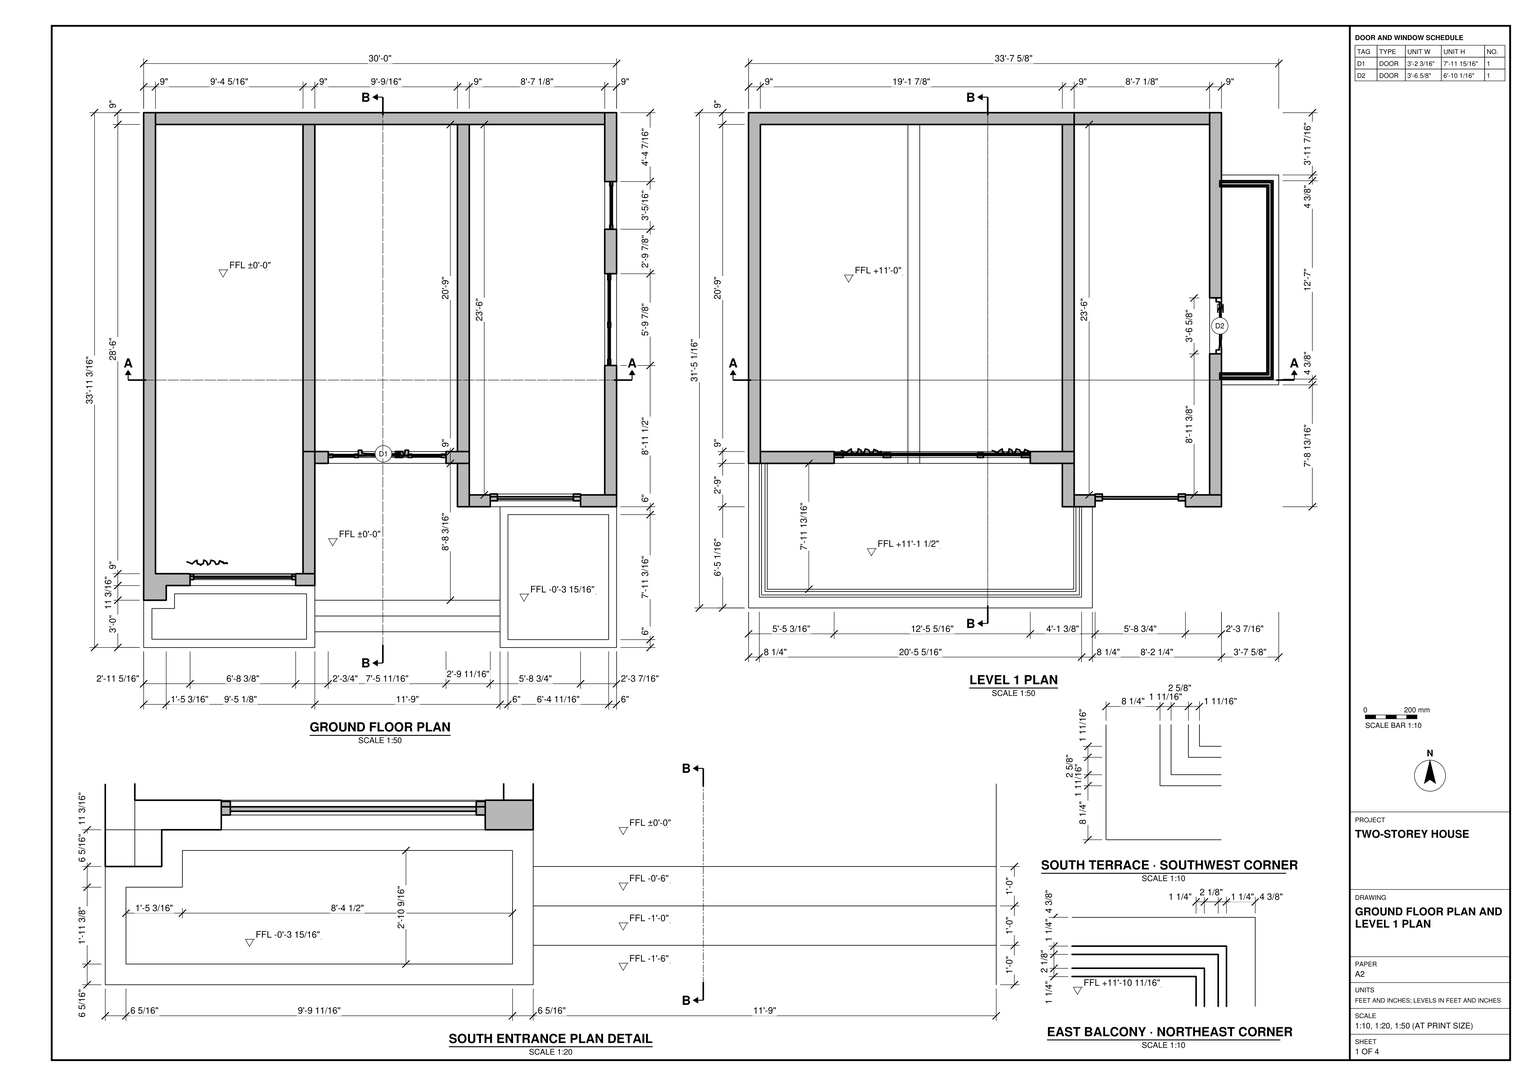
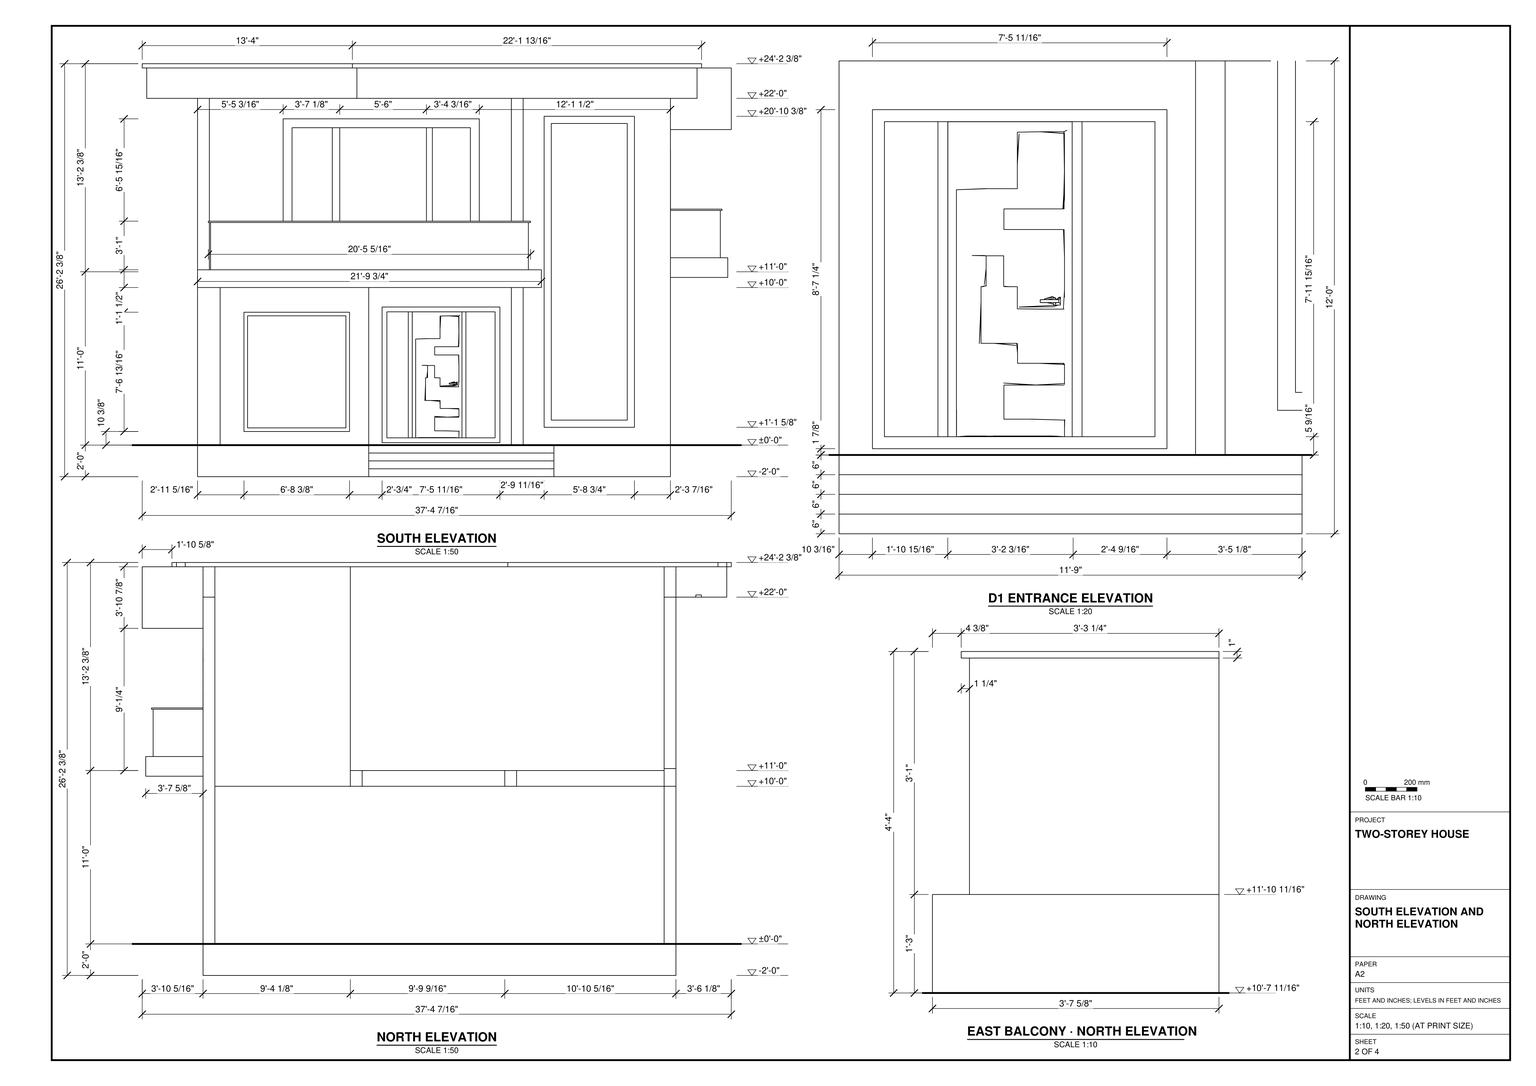
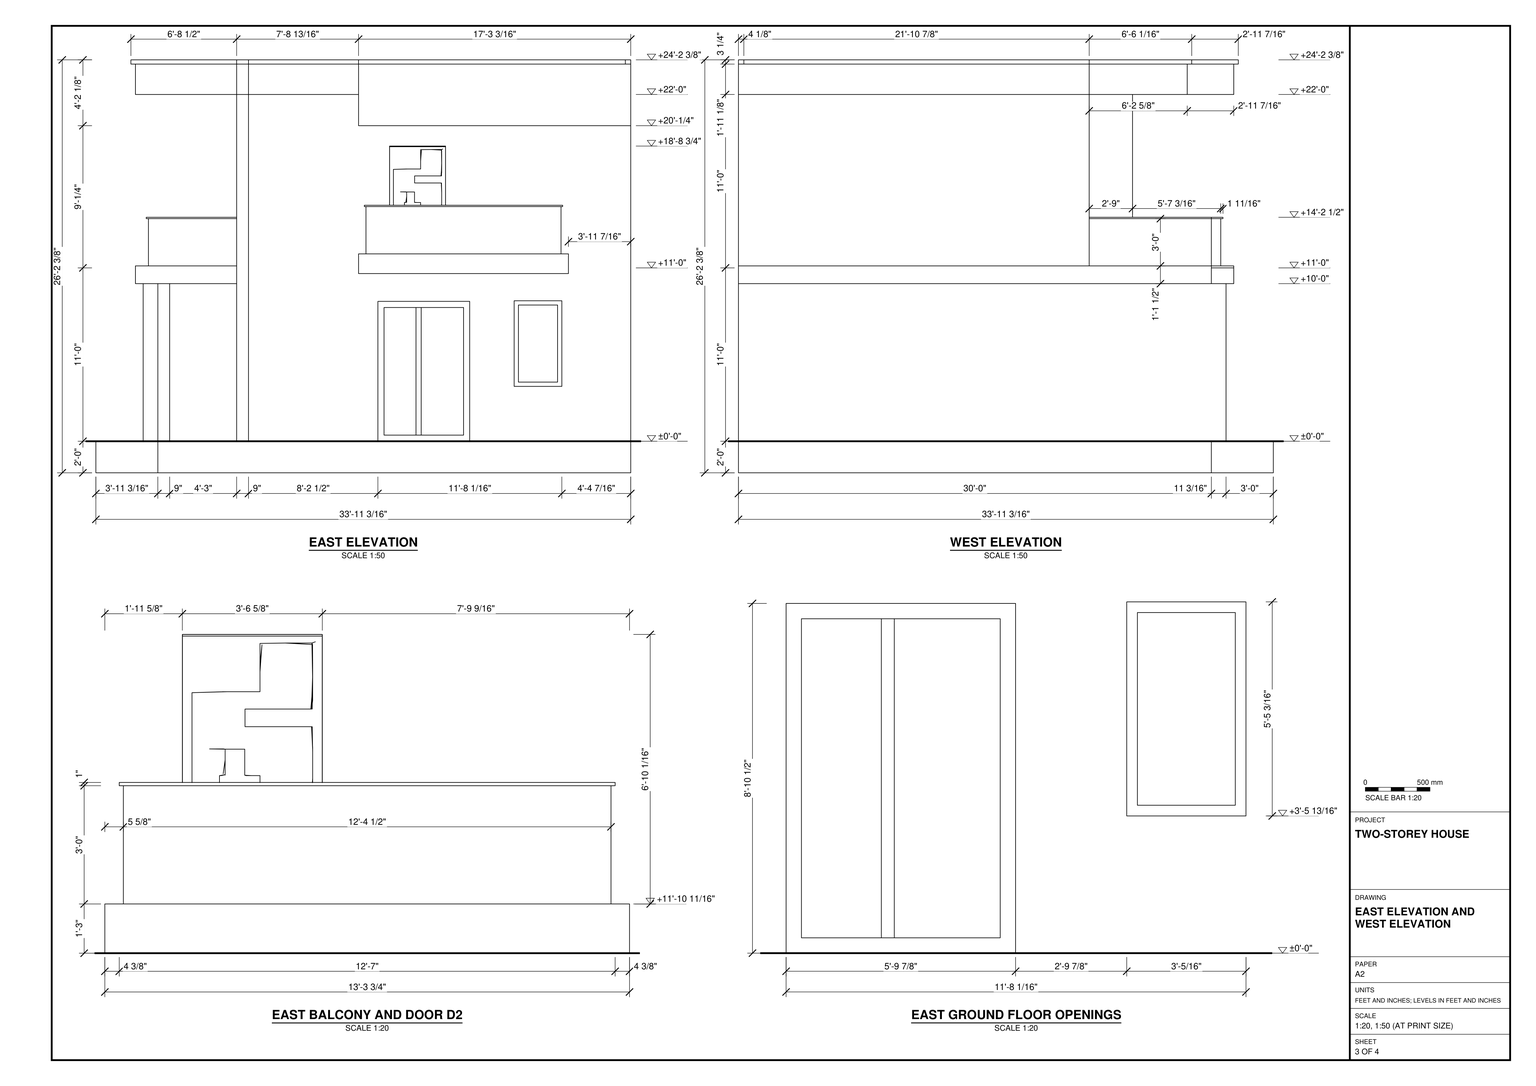
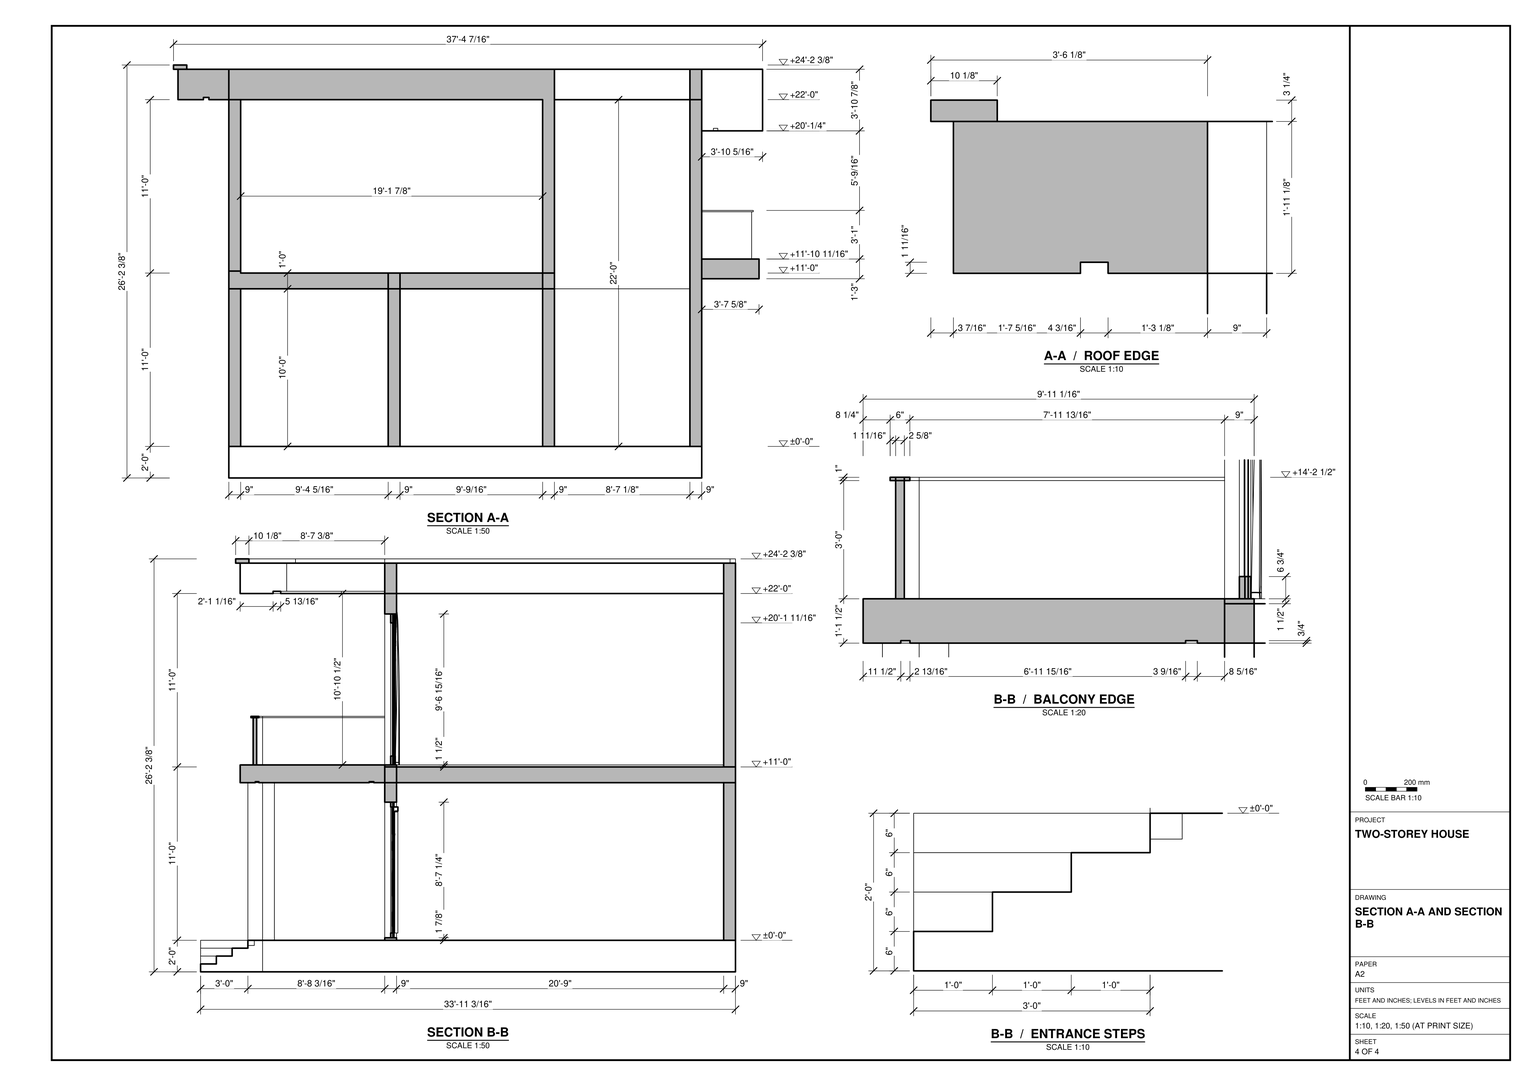
Build the house in SketchUp from task_files/diagram_01.pdf. Work in feet and inches. The overall model extents are 37'-4 7/16" east to west, 33'-11 3/16" north to south and 26'-2 3/8" from the bottom of the base to the top of the roof. Set the ground floor at ±0'-0" and the upper floor at +11'-0".

Use the plans to lay out the base, floor slabs and walls. Follow the 9" wall thicknesses where indicated. On the ground floor, run the partitions north to south and set the central entrance back between the flanking bays. Model the broad approach steps, entrance door and side panels. On the upper floor, set the wall back from the south slab edge to form the terrace above the entrance. Include its guard and the separate projecting east balcony with its guard and access door. Use the elevations to place the framed openings, including the tall opening at the east end of the south facade and the two differently sized openings below the east balcony. Finish the shell with the overhanging flat roof and its fascia profile.

Keep walls, slabs and roof as separate groups or components, and group each furniture or joinery piece separately if shown. Use components for repeated parts. Decor and loose items may be any suitable library components. Save one SketchUp model as output_files/two_storey_house_with_a_south_terrace_and_east_balcony.skp.

# SketchUp Ruby script. Lengths in inches.
U = 1.inch
M = Sketchup.active_model
def pt(a) = Geom::Point3d.new(a.map { |v| v * U })
def face(e, loops, mat)
  f = e.add_face(loops[0].map { |a| pt(a) })
  loops[1..].each { |l| e.add_face(l.map { |a| pt(a) }).erase! }
  f.material = f.back_material = mat if mat
  f
end
# faces: each face lists its corners as indices into pts; further lists are holes
def faces(e, pts, list, mat = nil) = list.each { |f| face(e, (f[0].is_a?(Array) ? f : [f]).map { |l| l.map { |i| pts[i] } }, mat) }
# xy, xz, yz: faces in a plane at the given z, y or x. An outline is a flat list of corners, or four numbers for a rectangle; further outlines are holes
def ring(l) = l.size == 4 ? [[l[0], l[1]], [l[2], l[1]], [l[2], l[3]], [l[0], l[3]]] : l.each_slice(2).to_a
def flat(e, list, mat, &to3) = list.each { |f| face(e, (f[0].is_a?(Array) ? f : [f]).map { |l| ring(l).map { |u, v| to3.(u, v) } }, mat) }
def xy(e, z, list, mat = nil) = flat(e, list, mat) { |x, y| [x, y, z] }
def xz(e, y, list, mat = nil) = flat(e, list, mat) { |x, z| [x, y, z] }
def yz(e, x, list, mat = nil) = flat(e, list, mat) { |y, z| [x, y, z] }
def lines(e, pts, list) = list.each { |a, b| e.add_line(pt(pts[a]), pt(pts[b])) }
# prism: a flat outline (further loops are holes) pulled along v
def prism(e, loops, v, mat = nil)
  f = face(e, loops, mat); d = Geom::Vector3d.new(v.map { |x| x * U })
  f.pushpull(f.normal.samedirection?(d) ? d.length : -d.length)
end
def box(e, o, s, mat = nil) = prism(e, [[o, [o[0] + s[0], o[1], o[2]], [o[0] + s[0], o[1] + s[1], o[2]], [o[0], o[1] + s[1], o[2]]]], [0, 0, s[2]], mat)
def at(x, y, z, deg = 0) = Geom::Transformation.translation(pt([x, y, z])) * Geom::Transformation.rotation(ORIGIN, Z_AXIS, deg.degrees)
def axes(o, x, y, z) = Geom::Transformation.new([*x, 0, *y, 0, *z, 0, *pt(o).to_a, 1])
def part(name) = M.definitions.add(name)
# library, detail: a bought-in or finely detailed component or shape, given as its bounding box
def library(name, o, s) = part(name).tap { |d| box(d.entities, o, s) }
def detail(e, o, s) = box(e.add_group.entities, o, s)
def put(e, d, t, mat = nil) = e.add_instance(d, t).tap { |i| i.material = mat if mat }
def group(e, t, mat = nil) = e.add_group.tap { |g| g.transformation = t; g.material = mat if mat }.entities
root = M.entities
M.materials.add("Emissive").color = [236, 234, 181]
M.materials.add("Glass Smoked Frosted 001").color = [243, 240, 240]
M.materials["Glass Smoked Frosted 001"].alpha = 0.1
M.materials.add("[Color M01]").color = [226, 226, 226]
M.materials.add("[Color M07]").color = [58, 58, 58]
M.materials.add("[Stone Vein Gray]").color = [166, 165, 165]
c1 = library("Curtains 004",[-15.59,-2.26,0],[31.18,4.52,116.91])
c2 = library("Door 243 069",[-19.08,-2.76,0],[38.16,5.52,82.08])
xy(root,-24,[[42.125,0,402.125,47.1875],[42.125,47.1875,402.125,407.1875]])
xy(root,-18,[[172.4375,0,313.43,12]],"[Stone Vein Gray]")
xy(root,-12,[[172.4375,12,313.43,24]],"[Stone Vein Gray]")
xy(root,-6,[[172.4375,24,313.43,36]],"[Stone Vein Gray]")
xy(root,-3.9375,[[319.44,6.01,396.11,101.17]])
xy(root,-3.9375,[[48.43,6.3,166.14,6.3,166.14,40.89,65.61,40.89,65.61,29.7,48.43,29.7]],"[Color M01]")
xy(root,0,[[[313.43,0,402.125,107.1875],[319.44,6.01,396.11,101.17]],[42.125,36,51.125,47.1875],[51.125,36,59.3125,47.1875],[42.125,47.1875,51.125,407.1875],[51.125,47.1875,172.4375,56.1875],
  [51.125,56.1875,163.4375,398.1875],[163.4375,56.1875,172.4375,149.1875],[163.4375,56.1875,172.4375,56.1875,172.4375,140.1875,281,140.1875,281,107.1875,290,107.1875,290,398.1875,163.4375,398.1875],[281,107.1875,290,140.1875],[290,107.1875,393.125,116.1875],
  [393.125,107.1875,402.125,116.1875],[290,116.1875,393.125,398.1875],[393.125,116.1875,402.125,214.71],[172.4375,140.1875,290,149.1875],[163.4375,149.1875,172.4375,398.1875],
  [172.4375,149.1875,281,398.1875],[281,149.1875,290,398.1875],[393.125,214.71,395.4375,284.58],[395.4375,214.71,397.625,284.58],[397.625,214.71,402.125,284.58],
  [393.125,284.58,402.125,407.1875],[51.125,398.1875,393.125,407.1875]])
xy(root,0,[[[42.125,0,172.4375,0,172.4375,47.1875,59.3125,47.1875,59.3125,36,42.125,36],[48.43,6.3,48.43,29.7,65.61,29.7,65.61,40.89,166.14,40.89,166.14,6.3]]],"[Color M01]")
xy(root,0,[[395.4375,214.71,396.3125,284.58],[396.3125,214.71,397.625,284.58]],"[Color M07]")
xy(root,0,[[172.4375,36,313.43,36,313.43,107.1875,281,107.1875,281,140.1875,172.4375,140.1875]],"[Stone Vein Gray]")
xy(root,1.91,[[182.61,140.1875,272.3,144.6875],[182.61,144.6875,272.3,146.4375],[182.61,146.4375,272.3,147.1875],[182.61,147.1875,272.3,149.1875]])
xy(root,4.67,[[395.4375,243.71,397.625,247.65]])
xy(root,4.67,[[395.4375,219.38,397.25,243.71],[397.25,219.38,397.625,243.71],[395.4375,247.65,397.25,279.91],[397.25,247.65,397.625,279.91]],"[Color M07]")
xy(root,5.56,[[202.55,144.6875,205.56,147.1875],[243.43,144.6875,246.43,147.1875]])
xy(root,5.56,[[186.26,144.6875,202.55,145.4375],[205.56,144.6875,243.43,145.4375],[246.43,144.6875,268.64,145.4375],[186.26,145.4375,202.55,147.1875],[205.56,145.4375,243.43,147.1875],
  [246.43,145.4375,268.64,147.1875]],"[Color M07]")
xy(root,10.38,[[77.46,47.1875,157.83,51.6875],[77.46,51.6875,157.83,54.1875],[77.46,54.1875,157.83,55.8125],[77.46,55.8125,157.83,56.1875]])
xy(root,13.14,[[80.21,51.6875,155.08,52.8125],[80.21,52.8125,155.08,55.8125]],"[Color M07]")
xy(root,13.6,[[305.97,107.1875,374.72,111.6875],[305.97,111.6875,374.72,114.8125],[305.97,114.8125,374.72,116.1875],[305.97,116.1875,374.72,116.875]])
xy(root,19.06,[[311.43,111.6875,369.26,113],[311.43,113,369.26,116.875]],"[Color M07]")
xy(root,41.78,[[393.125,318.43,397,354.74],[399.1875,318.43,402.125,354.74]])
xy(root,41.78,[[397,318.43,397.625,354.74],[397.625,318.43,399.1875,354.74]],"[Color M07]")
xy(root,45.04,[[397,321.68,398.8125,351.49],[398.8125,321.68,399.1875,351.49]],"[Color M07]")
xy(root,98.44,[[80.21,51.6875,155.08,52.8125],[80.21,52.8125,155.08,55.8125]],"[Color M07]")
xy(root,101.2,[[77.46,47.1875,157.83,51.6875],[77.46,55.8125,157.83,56.1875]])
xy(root,101.2,[[77.46,51.6875,157.83,54.1875],[77.46,54.1875,157.83,55.8125]],"[Color M07]")
xy(root,101.5,[[202.55,144.6875,205.56,147.1875],[243.43,144.6875,246.43,147.1875]])
xy(root,101.5,[[186.26,144.6875,202.55,145.4375],[205.56,144.6875,243.43,145.4375],[246.43,144.6875,268.64,145.4375],[186.26,145.4375,202.55,147.1875],[205.56,145.4375,243.43,147.1875],
  [246.43,145.4375,268.64,147.1875]],"[Color M07]")
xy(root,101.83,[[395.4375,243.71,397.625,247.65]])
xy(root,101.83,[[395.4375,219.38,397.25,243.71],[397.25,219.38,397.625,243.71],[395.4375,247.65,397.25,279.91],[397.25,247.65,397.625,279.91]],"[Color M07]")
xy(root,103.72,[[397,321.68,398.8125,351.49],[398.8125,321.68,399.1875,351.49]],"[Color M07]")
xy(root,105.16,[[182.61,140.1875,272.3,144.6875],[182.61,147.1875,272.3,149.1875]])
xy(root,105.16,[[182.61,144.6875,272.3,146.4375],[182.61,146.4375,272.3,147.1875]],"[Color M07]")
xy(root,106.5,[[393.125,214.71,395.4375,284.58],[397.625,214.71,402.125,284.58]])
xy(root,106.5,[[395.4375,214.71,396.3125,284.58],[396.3125,214.71,397.625,284.58]],"[Color M07]")
xy(root,106.97,[[393.125,318.43,397,354.74],[399.1875,318.43,402.125,354.74]])
xy(root,106.97,[[397,318.43,397.625,354.74],[397.625,318.43,399.1875,354.74]],"[Color M07]")
xy(root,120,[[42.125,30.125,51.125,36],[51.125,30.125,59.3125,36],[59.3125,30.125,59.3125,41.59,297.1875,41.59,297.1875,107.1875,303.875,107.1875,303.875,30.125],[42.125,36,51.125,47.1875],[51.125,36,59.3125,47.1875],
  [59.3125,44.39,59.3125,47.1875,172.4375,47.1875,172.4375,140.1875,281,140.1875,281,131.89,176.45,131.89,176.45,44.39],[178.54,44.39,178.54,128.32,281,128.32,281,107.1875,293.59,107.1875,293.59,44.39],[42.125,47.1875,51.125,407.1875],[51.125,47.1875,172.4375,56.1875],[51.125,56.1875,163.4375,398.1875],
  [163.4375,56.1875,172.4375,149.1875],[172.4375,140.1875,290,149.1875],[163.4375,149.1875,172.4375,398.1875],[172.4375,149.1875,281,398.1875],[281,149.1875,290,398.1875],
  [51.125,398.1875,163.4375,407.1875],[163.4375,398.1875,172.4375,407.1875],[172.4375,398.1875,281,407.1875],[281,398.1875,290,407.1875],[290,398.1875,393.125,407.1875]])
xy(root,120.75,[[59.3125,41.59,59.3125,44.39,293.59,44.39,293.59,107.1875,297.1875,107.1875,297.1875,41.59],[176.45,44.39,178.54,131.89],[178.54,128.32,281,131.89]])
xy(root,127.66,[[402.125,199.99,445.75,359.75]])
xy(root,132,[[51.125,140.1875,163.4375,149.1875],[163.4375,140.1875,172.4375,149.1875],[172.4375,140.1875,290,149.1875],[51.125,149.1875,163.4375,398.1875],[163.4375,149.1875,172.4375,398.1875],
  [172.4375,149.1875,281,398.1875],[281,149.1875,290,398.1875],[51.125,398.1875,163.4375,407.1875],[163.4375,398.1875,172.4375,407.1875],[172.4375,398.1875,281,407.1875],
  [281,398.1875,290,407.1875]])
xy(root,133.5,[[52.03,40.03,52.03,140.1875,54.67,140.1875,54.67,42.67,291.33,42.67,291.33,107.1875,293.97,107.1875,293.97,40.03],[54.67,42.67,291.33,42.67,291.33,107.1875,281,107.1875,281,140.1875,54.67,140.1875],[42.125,140.1875,51.125,407.1875],[107.28,140.1875,163.4375,144.6875],[163.4375,140.1875,172.4375,144.6875],
  [172.4375,140.1875,256.59,144.6875],[107.28,148.1875,163.4375,149.1875],[163.4375,148.1875,172.4375,149.1875],[172.4375,148.1875,256.59,149.1875]])
xy(root,133.5,[[42.125,30.125,303.875,30.125,303.875,107.1875,293.97,107.1875,293.97,40.03,52.03,40.03,52.03,140.1875,42.125,140.1875]],"[Color M01]")
xy(root,133.5,[[107.28,144.6875,163.4375,146.375],[163.4375,144.6875,172.4375,146.375],[172.4375,144.6875,256.59,146.375],[107.28,146.375,163.4375,147.375],[163.4375,146.375,172.4375,147.375],
  [172.4375,146.375,256.59,147.375],[107.28,147.375,163.4375,148.1875],[163.4375,147.375,172.4375,148.1875],[172.4375,147.375,256.59,148.1875]],"[Color M07]")
xy(root,140.27,[[114.05,144.6875,144.7,146.25],[144.7,144.6875,150.39,146.375],[150.39,144.6875,163.4375,146.25],[163.4375,144.6875,172.4375,146.25],[172.4375,144.6875,216.38,146.25],
  [216.38,144.6875,220.9,146.375],[220.9,144.6875,249.82,146.25],[114.05,146.25,144.7,146.375],[150.39,146.25,163.4375,146.375],[163.4375,146.25,172.4375,146.375],
  [172.4375,146.25,216.38,146.375],[220.9,146.25,249.82,146.375],[114.05,146.375,144.7,148.1875],[144.7,146.375,150.39,148.1875],[150.39,146.375,163.4375,148.1875],
  [163.4375,146.375,172.4375,148.1875],[172.4375,146.375,216.38,148.1875],[216.38,146.375,220.9,148.1875],[220.9,146.375,249.82,148.1875]],"[Color M07]")
xy(root,142.66,[[402.125,199.99,445.75,199.99,445.75,359.75,402.125,359.75,402.125,354.11,440.11,354.11,440.11,205.625,402.125,205.625],[402.125,205.625,402.125,207.73,438.01,207.73,438.01,352.01,402.125,352.01,402.125,354.11,440.11,354.11,440.11,205.625],[402.125,207.73,438.01,352.01],[393.125,223.58,402.125,266.21]])
xy(root,169.5,[[52.03,40.03,52.03,140.1875,54.67,140.1875,54.67,42.67,291.33,42.67,291.33,107.1875,293.97,107.1875,293.97,40.03]])
xy(root,169.5,[[[50.34,38.34,50.34,141.87,56.35,141.87,56.35,44.35,289.65,44.35,289.65,108.87,295.66,108.87,295.66,38.34],[52.03,40.03,293.97,40.03,293.97,107.1875,291.33,107.1875,291.33,42.67,54.67,42.67,54.67,140.1875,52.03,140.1875]]],"[Color M07]")
xy(root,170.5,[[[50.34,38.34,295.66,38.34,295.66,108.87,289.65,108.87,289.65,44.35,56.35,44.35,56.35,141.87,50.34,141.87],[52.03,40.03,52.03,140.1875,54.67,140.1875,54.67,42.67,291.33,42.67,291.33,107.1875,293.97,107.1875,293.97,40.03]],[52.03,40.03,293.97,40.03,293.97,107.1875,291.33,107.1875,291.33,42.67,54.67,42.67,54.67,140.1875,52.03,140.1875]],"[Color M07]")
xy(root,178.66,[[402.125,205.625,402.125,207.73,438.01,207.73,438.01,352.01,402.125,352.01,402.125,354.11,440.11,354.11,440.11,205.625]])
xy(root,178.66,[[[400.86,204.36,400.86,208.99,436.75,208.99,436.75,350.74,400.86,350.74,400.86,355.37,441.37,355.37,441.37,204.36],[402.125,205.625,440.11,205.625,440.11,354.11,402.125,354.11,402.125,352.01,438.01,352.01,438.01,207.73,402.125,207.73]]],"[Color M07]")
xy(root,179.66,[[[400.86,204.36,441.37,204.36,441.37,355.37,400.86,355.37,400.86,350.74,436.75,350.74,436.75,208.99,400.86,208.99],[402.125,205.625,402.125,207.73,438.01,207.73,438.01,352.01,402.125,352.01,402.125,354.11,440.11,354.11,440.11,205.625]],[402.125,205.625,440.11,205.625,440.11,354.11,402.125,354.11,402.125,352.01,438.01,352.01,438.01,207.73,402.125,207.73]],"[Color M07]")
xy(root,224.22,[[393.125,223.58,402.125,266.21]])
xy(root,240.25,[[[402.125,199.99,448.4375,407.1875],[410.99,214.21,414.36,392.96]]])
xy(root,241.67,[[114.05,144.6875,144.7,146.25],[144.7,144.6875,150.39,146.375],[150.39,144.6875,216.38,146.25],[216.38,144.6875,220.9,146.375],[220.9,144.6875,249.82,146.25],
  [114.05,146.25,144.7,146.375],[150.39,146.25,216.38,146.375],[220.9,146.25,249.82,146.375],[114.05,146.375,144.7,148.1875],[144.7,146.375,150.39,148.1875],
  [150.39,146.375,216.38,148.1875],[216.38,146.375,220.9,148.1875],[220.9,146.375,249.82,148.1875]],"[Color M07]")
xy(root,242.1875,[[410.99,214.21,414.36,392.96]])
xy(root,244.88,[[311.43,111.6875,369.26,113],[311.43,113,369.26,116.875]],"[Color M07]")
xy(root,248.4375,[[107.28,140.1875,256.59,144.6875],[107.28,148.1875,256.59,149.1875]])
xy(root,248.4375,[[107.28,144.6875,256.59,146.375],[107.28,146.375,256.59,147.375],[107.28,147.375,256.59,148.1875]],"[Color M07]")
xy(root,250.35,[[305.97,107.1875,374.72,111.6875]])
xy(root,250.35,[[305.97,111.6875,374.72,114.8125],[305.97,114.8125,374.72,116.1875],[305.97,116.1875,374.72,116.875]],"[Color M07]")
xy(root,264,[[163.4375,30.125,163.4375,65.5625,3.4375,65.5625,3.4375,407.1875,22.78,407.1875,22.78,102.6875,208.22,102.6875,208.22,55.1875,340.91,55.1875,340.91,107.1875,402.125,107.1875,402.125,199.99,422.375,199.99,422.375,30.125],[212.86,61,212.86,107.1875,26.99,107.1875,26.99,407.1875,42.125,407.1875,42.125,140.1875,281,140.1875,281,107.1875,335.55,107.1875,335.55,61],[281,107.1875,290,140.1875],[290,107.1875,402.125,116.1875],[290,116.1875,393.125,398.1875],
  [393.125,116.1875,402.125,199.99],[42.125,140.1875,51.125,407.1875],[51.125,140.1875,163.4375,149.1875],[163.4375,140.1875,172.4375,149.1875],[172.4375,140.1875,290,149.1875],
  [51.125,149.1875,281,398.1875],[393.125,199.99,402.125,407.1875]])
xy(root,265.6875,[[208.22,55.1875,208.22,102.6875,22.78,102.6875,22.78,407.1875,26.99,407.1875,26.99,107.1875,212.86,107.1875,212.86,61,335.55,61,335.55,107.1875,340.91,107.1875,340.91,55.1875]])
xy(root,287.125,[[163.4375,30.125,163.4375,65.5625,3.4375,65.5625,3.4375,403.0625,10.11,403.0625,10.11,72.24,170.11,72.24,170.11,36.8,415.7,36.8,415.7,199.99,422.375,199.99,422.375,30.125],[281,107.1875,290,140.1875],[290,107.1875,402.125,116.1875],[290,116.1875,393.125,398.1875],[42.125,140.1875,51.125,140.1875,51.125,149.1875,281,149.1875,281,398.1875,51.125,398.1875,51.125,407.1875,42.125,407.1875],
  [51.125,140.1875,163.4375,149.1875],[163.4375,140.1875,172.4375,149.1875],[172.4375,140.1875,290,149.1875],[281,149.1875,290,398.1875],[393.125,199.99,402.125,407.1875],
  [402.125,199.99,448.4375,407.1875],[51.125,398.1875,290,407.1875],[290,398.1875,393.125,407.1875],[0,403.0625,3.4375,407.1875],[3.4375,403.0625,10.11,407.1875]])
xy(root,287.125,[[160,26.6875,160,62.125,0,62.125,0,403.0625,3.4375,403.0625,3.4375,65.5625,163.4375,65.5625,163.4375,30.125,422.375,30.125,422.375,199.99,425.8125,199.99,425.8125,26.6875],[170.11,36.8,415.7,36.8,415.7,199.99,393.125,199.99,393.125,116.1875,402.125,116.1875,402.125,107.1875,281,107.1875,281,140.1875,42.125,140.1875,42.125,407.1875,10.11,407.1875,10.11,72.24,170.11,72.24]],"[Color M01]")
xy(root,290.375,[[0,403.0625,3.4375,407.1875],[3.4375,403.0625,10.11,407.1875]])
xy(root,290.375,[[160,26.6875,425.8125,26.6875,425.8125,199.99,415.7,199.99,415.7,36.8,170.11,36.8,170.11,72.24,10.11,72.24,10.11,403.0625,0,403.0625,0,62.125,160,62.125]],"[Color M01]")
xz(root,0,[[42.125,-24,172.4375,0],[313.43,-24,402.125,0]],"[Color M01]")
xz(root,0,[[172.4375,-24,313.43,-18]],"[Stone Vein Gray]")
xz(root,6.01,[[319.44,-3.9375,396.11,0]])
xz(root,6.3,[[48.43,-3.9375,166.14,0]],"[Color M01]")
xz(root,12,[[172.4375,-18,313.43,-12]],"[Stone Vein Gray]")
xz(root,24,[[172.4375,-12,313.43,-6]],"[Stone Vein Gray]")
xz(root,26.6875,[[160,287.125,425.8125,290.375]],"[Color M01]")
xz(root,29.7,[[48.43,-3.9375,51.125,0],[51.125,-3.9375,65.61,0]],"[Color M01]")
xz(root,30.125,[[42.125,120,303.875,133.5],[163.4375,264,422.375,287.125]],"[Color M01]")
xz(root,36,[[42.125,0,59.3125,120]],"[Color M01]")
xz(root,36,[[172.4375,-6,313.43,0]],"[Stone Vein Gray]")
xz(root,36.8,[[170.11,287.125,415.7,290.375]])
xz(root,38.34,[[50.34,169.5,295.66,170.5]],"[Color M07]")
xz(root,40.03,[[52.03,169.5,293.97,170.5]])
xz(root,40.03,[[52.03,133.5,293.97,169.5]],"Glass Smoked Frosted 001")
xz(root,40.89,[[65.61,-3.9375,166.14,0]],"[Color M01]")
xz(root,41.59,[[59.3125,120,297.1875,120.75]],"Emissive")
xz(root,42.67,[[54.67,169.5,291.33,170.5]])
xz(root,42.67,[[54.67,133.5,291.33,169.5]],"Glass Smoked Frosted 001")
xz(root,44.35,[[56.35,169.5,289.65,170.5]],"[Color M07]")
xz(root,44.39,[[59.3125,120,176.45,120.75],[178.54,120,293.59,120.75]],"Emissive")
xz(root,47.1875,[[42.125,120,51.125,132],[51.125,120,59.3125,132],[59.3125,120,172.4375,132]])
xz(root,47.1875,[[[59.3125,0,172.4375,120],[77.46,10.38,157.83,101.2]]],"[Color M01]")
xz(root,51.6875,[[[77.46,10.38,157.83,101.2],[80.21,13.14,155.08,98.44]]],"[Color M07]")
xz(root,52.8125,[[80.21,13.14,155.08,98.44]],"Glass Smoked Frosted 001")
xz(root,54.1875,[[77.46,10.38,157.83,101.2]],"Glass Smoked Frosted 001")
xz(root,55.1875,[[208.22,264,340.91,265.6875]],"Emissive")
xz(root,55.8125,[[[77.46,10.38,157.83,101.2],[80.21,13.14,155.08,98.44]]],"[Color M07]")
xz(root,56.1875,[[[51.125,0,163.4375,120],[77.46,10.38,157.83,101.2]],[163.4375,0,172.4375,120]])
xz(root,61,[[212.86,264,335.55,265.6875]],"Emissive")
xz(root,62.125,[[0,287.125,160,290.375]],"[Color M01]")
xz(root,65.5625,[[3.4375,264,163.4375,287.125]],"[Color M01]")
xz(root,72.24,[[10.11,287.125,170.11,290.375]])
xz(root,101.17,[[319.44,-3.9375,393.125,0],[393.125,-3.9375,396.11,0]])
xz(root,102.6875,[[22.78,264,208.22,265.6875]],"Emissive")
xz(root,107.1875,[[281,120,290,132],[290,120,290,132,303.875,132,303.875,120,297.1875,120,297.1875,120.75,293.59,120.75,293.59,120],[281,132,290,133.5],[290,132,303.875,133.5],[281,133.5,290,264],
  [291.33,133.5,293.97,169.5],[291.33,169.5,293.97,170.5],[281,264,290,287.125],[290,264,290,287.125,402.125,287.125,402.125,264,340.91,264,340.91,265.6875,335.55,265.6875,335.55,264],[335.55,264,340.91,265.6875]])
xz(root,107.1875,[[26.99,264,212.86,265.6875]],"Emissive")
xz(root,107.1875,[[281,0,290,120],[[290,0,402.125,0,402.125,264,290,264,290,133.5,291.33,133.5,291.33,170.5,293.97,170.5,293.97,133.5,303.875,133.5,303.875,120,297.1875,120,297.1875,120.75,293.59,120.75,293.59,120,290,120],[305.97,13.6,374.72,250.35]]],"[Color M01]")
xz(root,108.87,[[289.65,169.5,295.66,170.5]])
xz(root,111.6875,[[[305.97,13.6,374.72,250.35],[311.43,19.06,369.26,244.88]]],"[Color M07]")
xz(root,113,[[311.43,19.06,369.26,244.88]],"Glass Smoked Frosted 001")
xz(root,114.8125,[[305.97,13.6,374.72,250.35]],"Glass Smoked Frosted 001")
xz(root,116.1875,[[[290,0,393.125,264],[305.97,13.6,374.72,250.35]],[393.125,0,402.125,264],[290,264,393.125,287.125],[393.125,264,402.125,287.125]])
xz(root,116.875,[[[305.97,13.6,374.72,250.35],[311.43,19.06,369.26,244.88]]],"[Color M07]")
xz(root,128.32,[[178.54,120,281,120.75]],"Emissive")
xz(root,131.89,[[176.45,120,178.54,120.75],[178.54,120,281,120.75]],"Emissive")
xz(root,140.1875,[[281,0,290,120],[172.4375,120,281,132],[281,120,290,132],[51.125,132,163.4375,133.5],[163.4375,132,172.4375,133.5],
  [172.4375,132,281,133.5],[281,132,290,264],[52.03,133.5,54.67,169.5],[52.03,169.5,54.67,170.5],[42.125,264,51.125,287.125],
  [51.125,264,163.4375,287.125],[163.4375,264,172.4375,287.125],[172.4375,264,281,287.125],[281,264,290,287.125]])
xz(root,140.1875,[[[172.4375,0,281,120],[182.61,1.91,272.3,105.16]],[42.125,133.5,51.125,264],[51.125,133.5,52.03,133.5,52.03,170.5,54.67,170.5,54.67,133.5,107.28,133.5,107.28,248.4375,256.59,248.4375,256.59,133.5,281,133.5,281,264,51.125,264]],"[Color M01]")
xz(root,141.87,[[50.34,169.5,56.35,170.5]])
xz(root,144.6875,[[[182.61,1.91,272.3,105.16],[186.26,5.56,268.64,101.5]],[202.55,5.56,205.56,101.5],[243.43,5.56,246.43,101.5],[[107.28,133.5,256.59,248.4375],[114.05,140.27,249.82,241.67]],[144.7,140.27,150.39,241.67],
  [216.38,140.27,220.9,241.67]],"[Color M07]")
xz(root,145.4375,[[186.26,5.56,202.55,101.5],[246.43,5.56,268.64,101.5]],"Glass Smoked Frosted 001")
xz(root,146.25,[[114.05,140.27,144.7,241.67],[150.39,140.27,216.38,241.67],[220.9,140.27,249.82,241.67]],"Glass Smoked Frosted 001")
xz(root,146.375,[[[107.28,133.5,256.59,248.4375],[114.05,140.27,249.82,241.67]],[144.7,140.27,150.39,241.67],[216.38,140.27,220.9,241.67]],"[Color M07]")
xz(root,146.4375,[[182.61,1.91,272.3,105.16]],"Glass Smoked Frosted 001")
xz(root,147.1875,[[[182.61,1.91,272.3,105.16],[186.26,5.56,268.64,101.5]],[202.55,5.56,205.56,101.5],[243.43,5.56,246.43,101.5]],"[Color M07]")
xz(root,147.375,[[107.28,133.5,256.59,248.4375]],"Glass Smoked Frosted 001")
xz(root,148.1875,[[[107.28,133.5,256.59,248.4375],[114.05,140.27,249.82,241.67]],[144.7,140.27,150.39,241.67],[216.38,140.27,220.9,241.67]],"[Color M07]")
xz(root,149.1875,[[163.4375,0,172.4375,120],[[172.4375,0,281,120],[182.61,1.91,272.3,105.16]],[281,0,290,120],[163.4375,120,172.4375,132],[172.4375,120,281,132],
  [281,120,290,132],[51.125,132,51.125,264,163.4375,264,163.4375,248.4375,107.28,248.4375,107.28,133.5,163.4375,133.5,163.4375,132],[163.4375,132,172.4375,133.5],[172.4375,132,172.4375,133.5,256.59,133.5,256.59,248.4375,172.4375,248.4375,172.4375,264,281,264,281,132],[281,132,290,264],
  [163.4375,248.4375,172.4375,264],[51.125,264,163.4375,287.125],[163.4375,264,172.4375,287.125],[172.4375,264,281,287.125],[281,264,290,287.125]])
xz(root,199.99,[[402.125,127.66,445.75,142.66],[393.125,264,402.125,287.125],[402.125,264,422.375,287.125],[415.7,287.125,422.375,290.375],[422.375,287.125,425.8125,290.375]])
xz(root,199.99,[[402.125,240.25,448.4375,240.25,448.4375,287.125,422.375,287.125,422.375,264,402.125,264]],"[Color M01]")
xz(root,204.36,[[400.86,178.66,441.37,179.66]],"[Color M07]")
xz(root,205.625,[[402.125,178.66,440.11,179.66]])
xz(root,205.625,[[402.125,142.66,440.11,178.66]],"Glass Smoked Frosted 001")
xz(root,207.73,[[402.125,178.66,438.01,179.66]])
xz(root,207.73,[[402.125,142.66,438.01,178.66]],"Glass Smoked Frosted 001")
xz(root,208.99,[[400.86,178.66,436.75,179.66]],"[Color M07]")
xz(root,214.21,[[410.99,240.25,414.36,242.1875]],"Emissive")
xz(root,214.71,[[393.125,0,395.4375,106.5],[397.625,0,402.125,106.5]])
xz(root,214.71,[[395.4375,0,396.3125,106.5],[396.3125,0,397.625,106.5]],"[Color M07]")
xz(root,219.38,[[395.4375,4.67,397.25,101.83],[397.25,4.67,397.625,101.83]],"[Color M07]")
xz(root,223.58,[[393.125,142.66,402.125,224.22]])
xz(root,243.71,[[395.4375,4.67,397.25,101.83],[397.25,4.67,397.625,101.83]],"[Color M07]")
xz(root,247.65,[[395.4375,4.67,397.25,101.83],[397.25,4.67,397.625,101.83]],"[Color M07]")
xz(root,266.21,[[393.125,142.66,402.125,224.22]])
xz(root,279.91,[[395.4375,4.67,397.25,101.83],[397.25,4.67,397.625,101.83]],"[Color M07]")
xz(root,284.58,[[393.125,0,395.4375,106.5],[397.625,0,402.125,106.5]])
xz(root,284.58,[[395.4375,0,396.3125,106.5],[396.3125,0,397.625,106.5]],"[Color M07]")
xz(root,318.43,[[393.125,41.78,397,106.97],[399.1875,41.78,402.125,106.97]])
xz(root,318.43,[[397,41.78,397.625,106.97],[397.625,41.78,399.1875,106.97]],"[Color M07]")
xz(root,321.68,[[397,45.04,398.8125,103.72],[398.8125,45.04,399.1875,103.72]],"[Color M07]")
xz(root,350.74,[[400.86,178.66,436.75,179.66]],"[Color M07]")
xz(root,351.49,[[397,45.04,398.8125,103.72],[398.8125,45.04,399.1875,103.72]],"[Color M07]")
xz(root,352.01,[[402.125,178.66,438.01,179.66]])
xz(root,352.01,[[402.125,142.66,438.01,178.66]],"Glass Smoked Frosted 001")
xz(root,354.11,[[402.125,178.66,440.11,179.66]])
xz(root,354.11,[[402.125,142.66,440.11,178.66]],"Glass Smoked Frosted 001")
xz(root,354.74,[[393.125,41.78,397,106.97],[399.1875,41.78,402.125,106.97]])
xz(root,354.74,[[397,41.78,397.625,106.97],[397.625,41.78,399.1875,106.97]],"[Color M07]")
xz(root,355.37,[[400.86,178.66,441.37,179.66]],"[Color M07]")
xz(root,359.75,[[402.125,127.66,445.75,142.66]])
xz(root,392.96,[[410.99,240.25,414.36,242.1875]],"Emissive")
xz(root,398.1875,[[51.125,0,163.4375,120],[163.4375,0,172.4375,120],[172.4375,0,281,120],[281,0,290,120],[290,0,393.125,120],
  [290,120,393.125,264],[51.125,132,281,264],[281,132,290,287.125],[51.125,264,281,287.125]])
xz(root,403.0625,[[0,287.125,3.4375,290.375],[3.4375,287.125,10.11,290.375]])
xz(root,407.1875,[[42.125,-24,402.125,0],[42.125,0,51.125,120],[51.125,0,393.125,120],[393.125,0,402.125,264],[42.125,120,51.125,133.5],
  [51.125,120,163.4375,132],[163.4375,120,172.4375,132],[172.4375,120,281,132],[281,120,290,132],[290,120,393.125,287.125],
  [51.125,132,290,287.125],[42.125,133.5,51.125,264],[402.125,240.25,448.4375,287.125],[3.4375,264,3.4375,287.125,42.125,287.125,42.125,264,26.99,264,26.99,265.6875,22.78,265.6875,22.78,264],[42.125,264,51.125,287.125],
  [393.125,264,402.125,287.125],[0,287.125,3.4375,290.375],[3.4375,287.125,10.11,290.375]])
yz(root,0,[[62.125,287.125,140.1875,290.375],[140.1875,287.125,403.0625,290.375],[403.0625,287.125,407.1875,290.375]])
yz(root,3.4375,[[65.5625,264,140.1875,287.125],[140.1875,264,407.1875,287.125]],"[Color M01]")
yz(root,10.11,[[72.24,287.125,140.1875,290.375],[140.1875,287.125,403.0625,290.375],[403.0625,287.125,407.1875,290.375]])
yz(root,22.78,[[102.6875,264,407.1875,265.6875]],"Emissive")
yz(root,26.99,[[107.1875,264,407.1875,265.6875]],"Emissive")
yz(root,42.125,[[0,-24,47.1875,0],[140.1875,264,407.1875,287.125]])
yz(root,42.125,[[47.1875,-24,407.1875,0],[36,0,407.1875,120],[30.125,120,47.1875,132],[47.1875,120,407.1875,133.5],[30.125,132,47.1875,133.5],
  [140.1875,133.5,407.1875,264]],"[Color M01]")
yz(root,48.43,[[6.3,-3.9375,29.7,0]],"[Color M01]")
yz(root,50.34,[[38.34,169.5,47.1875,170.5],[47.1875,169.5,141.87,170.5]],"[Color M07]")
yz(root,51.125,[[56.1875,0,398.1875,120],[398.1875,0,407.1875,120],[398.1875,120,407.1875,132],[140.1875,132,149.1875,133.5],[149.1875,132,398.1875,133.5],
  [398.1875,132,407.1875,133.5],[140.1875,133.5,149.1875,264],[149.1875,133.5,398.1875,264],[140.1875,264,149.1875,287.125],[398.1875,264,407.1875,287.125]])
yz(root,52.03,[[40.03,169.5,47.1875,170.5],[47.1875,169.5,140.1875,170.5]])
yz(root,52.03,[[40.03,133.5,47.1875,169.5],[47.1875,133.5,140.1875,169.5]],"Glass Smoked Frosted 001")
yz(root,54.67,[[42.67,169.5,47.1875,170.5],[47.1875,169.5,140.1875,170.5]])
yz(root,54.67,[[42.67,133.5,47.1875,169.5],[47.1875,133.5,140.1875,169.5]],"Glass Smoked Frosted 001")
yz(root,56.35,[[44.35,169.5,47.1875,170.5],[47.1875,169.5,141.87,170.5]],"[Color M07]")
yz(root,59.3125,[[41.59,120,44.39,120.75]])
yz(root,59.3125,[[36,0,47.1875,120]],"[Color M01]")
yz(root,65.61,[[29.7,-3.9375,40.89,0]],"[Color M01]")
yz(root,77.46,[[47.1875,10.38,51.6875,101.2],[55.8125,10.38,56.1875,101.2]])
yz(root,77.46,[[51.6875,10.38,54.1875,101.2],[54.1875,10.38,55.8125,101.2]],"[Color M07]")
yz(root,80.21,[[51.6875,13.14,52.8125,98.44],[52.8125,13.14,55.8125,98.44]],"[Color M07]")
yz(root,107.28,[[140.1875,133.5,144.6875,248.4375],[148.1875,133.5,149.1875,248.4375]])
yz(root,107.28,[[144.6875,133.5,146.375,248.4375],[146.375,133.5,147.375,248.4375],[147.375,133.5,148.1875,248.4375]],"[Color M07]")
yz(root,114.05,[[144.6875,140.27,146.25,241.67],[146.25,140.27,146.375,241.67],[146.375,140.27,148.1875,241.67]],"[Color M07]")
yz(root,144.7,[[144.6875,140.27,146.25,241.67],[146.25,140.27,146.375,241.67],[146.375,140.27,148.1875,241.67]],"[Color M07]")
yz(root,150.39,[[144.6875,140.27,146.25,241.67],[146.25,140.27,146.375,241.67],[146.375,140.27,148.1875,241.67]],"[Color M07]")
yz(root,155.08,[[51.6875,13.14,52.8125,98.44],[52.8125,13.14,55.8125,98.44]],"[Color M07]")
yz(root,157.83,[[47.1875,10.38,51.6875,101.2],[55.8125,10.38,56.1875,101.2]])
yz(root,157.83,[[51.6875,10.38,54.1875,101.2],[54.1875,10.38,55.8125,101.2]],"[Color M07]")
yz(root,160,[[26.6875,287.125,62.125,290.375]],"[Color M01]")
yz(root,163.4375,[[56.1875,0,149.1875,120],[149.1875,0,398.1875,120],[149.1875,120,407.1875,132],[140.1875,264,149.1875,287.125]])
yz(root,163.4375,[[30.125,264,65.5625,287.125]],"[Color M01]")
yz(root,166.14,[[6.3,-3.9375,36,0],[36,-3.9375,40.89,0]],"[Color M01]")
yz(root,170.11,[[36.8,287.125,72.24,290.375]])
yz(root,172.4375,[[140.1875,0,149.1875,120],[149.1875,0,398.1875,120],[47.1875,120,56.1875,132],[56.1875,120,140.1875,132],[140.1875,120,149.1875,132],
  [149.1875,120,407.1875,132],[140.1875,264,149.1875,287.125]])
yz(root,172.4375,[[0,-18,12,-12],[0,-12,24,-6],[0,-6,36,0],[47.1875,0,56.1875,120],[56.1875,0,140.1875,120]],"[Color M01]")
yz(root,176.45,[[44.39,120,131.89,120.75]],"Emissive")
yz(root,178.54,[[44.39,120,128.32,120.75]],"Emissive")
yz(root,182.61,[[140.1875,1.91,144.6875,105.16],[147.1875,1.91,149.1875,105.16]])
yz(root,182.61,[[144.6875,1.91,146.4375,105.16],[146.4375,1.91,147.1875,105.16]],"[Color M07]")
yz(root,186.26,[[144.6875,5.56,145.4375,101.5],[145.4375,5.56,147.1875,101.5]],"[Color M07]")
yz(root,202.55,[[144.6875,5.56,145.4375,101.5],[145.4375,5.56,147.1875,101.5]],"[Color M07]")
yz(root,205.56,[[144.6875,5.56,145.4375,101.5],[145.4375,5.56,147.1875,101.5]],"[Color M07]")
yz(root,208.22,[[55.1875,264,102.6875,265.6875]],"Emissive")
yz(root,212.86,[[61,264,107.1875,265.6875]],"Emissive")
yz(root,216.38,[[144.6875,140.27,146.25,241.67],[146.25,140.27,146.375,241.67],[146.375,140.27,148.1875,241.67]],"[Color M07]")
yz(root,220.9,[[144.6875,140.27,146.25,241.67],[146.25,140.27,146.375,241.67],[146.375,140.27,148.1875,241.67]],"[Color M07]")
yz(root,243.43,[[144.6875,5.56,145.4375,101.5],[145.4375,5.56,147.1875,101.5]],"[Color M07]")
yz(root,246.43,[[144.6875,5.56,145.4375,101.5],[145.4375,5.56,147.1875,101.5]],"[Color M07]")
yz(root,249.82,[[144.6875,140.27,146.25,241.67],[146.25,140.27,146.375,241.67],[146.375,140.27,148.1875,241.67]],"[Color M07]")
yz(root,256.59,[[140.1875,133.5,144.6875,248.4375],[148.1875,133.5,149.1875,248.4375]])
yz(root,256.59,[[144.6875,133.5,146.375,248.4375],[146.375,133.5,147.375,248.4375],[147.375,133.5,148.1875,248.4375]],"[Color M07]")
yz(root,268.64,[[144.6875,5.56,145.4375,101.5],[145.4375,5.56,147.1875,101.5]],"[Color M07]")
yz(root,272.3,[[140.1875,1.91,144.6875,105.16],[147.1875,1.91,149.1875,105.16]])
yz(root,272.3,[[144.6875,1.91,146.4375,105.16],[146.4375,1.91,147.1875,105.16]],"[Color M07]")
yz(root,281,[[107.1875,0,107.1875,120,128.32,120,128.32,120.75,131.89,120.75,131.89,120,140.1875,120,140.1875,0],[149.1875,0,398.1875,120],[107.1875,120,107.1875,132,140.1875,132,140.1875,120,131.89,120,131.89,120.75,128.32,120.75,128.32,120],[149.1875,120,407.1875,132],[107.1875,132,140.1875,133.5],
  [149.1875,132,398.1875,264],[107.1875,133.5,140.1875,264],[107.1875,264,140.1875,287.125]])
yz(root,289.65,[[44.35,169.5,108.87,170.5]],"[Color M07]")
yz(root,290,[[107.1875,0,116.1875,264],[116.1875,0,140.1875,264],[140.1875,0,149.1875,120],[149.1875,0,398.1875,120],[140.1875,120,149.1875,132],
  [149.1875,120,398.1875,132],[398.1875,120,407.1875,132],[140.1875,132,149.1875,264],[149.1875,132,398.1875,264],[398.1875,132,407.1875,287.125],
  [107.1875,264,116.1875,287.125],[116.1875,264,140.1875,287.125],[140.1875,264,149.1875,287.125],[149.1875,264,398.1875,287.125]])
yz(root,291.33,[[42.67,169.5,107.1875,170.5]])
yz(root,291.33,[[42.67,133.5,107.1875,169.5]],"Glass Smoked Frosted 001")
yz(root,293.59,[[44.39,120,107.1875,120.75]],"Emissive")
yz(root,293.97,[[40.03,169.5,107.1875,170.5]])
yz(root,293.97,[[40.03,133.5,107.1875,169.5]],"Glass Smoked Frosted 001")
yz(root,295.66,[[38.34,169.5,108.87,170.5]],"[Color M07]")
yz(root,297.1875,[[41.59,120,107.1875,120.75]],"Emissive")
yz(root,303.875,[[30.125,120,107.1875,133.5]],"[Color M01]")
yz(root,305.97,[[107.1875,13.6,111.6875,250.35]])
yz(root,305.97,[[111.6875,13.6,114.8125,250.35],[114.8125,13.6,116.1875,250.35],[116.1875,13.6,116.875,250.35]],"[Color M07]")
yz(root,311.43,[[111.6875,19.06,113,244.88],[113,19.06,116.875,244.88]],"[Color M07]")
yz(root,313.43,[[0,-18,12,-12],[0,-12,24,-6],[0,-6,36,0]],"[Color M01]")
yz(root,319.44,[[6.01,-3.9375,36,0],[36,-3.9375,101.17,0]])
yz(root,335.55,[[61,264,107.1875,265.6875]],"Emissive")
yz(root,340.91,[[55.1875,264,107.1875,265.6875]],"Emissive")
yz(root,369.26,[[111.6875,19.06,113,244.88],[113,19.06,116.875,244.88]],"[Color M07]")
yz(root,374.72,[[107.1875,13.6,111.6875,250.35]])
yz(root,374.72,[[111.6875,13.6,114.8125,250.35],[114.8125,13.6,116.1875,250.35],[116.1875,13.6,116.875,250.35]],"[Color M07]")
yz(root,393.125,[[[116.1875,0,116.1875,264,398.1875,264,398.1875,0,284.58,0,284.58,106.5,214.71,106.5,214.71,0],[223.58,142.66,266.21,224.22],[318.43,41.78,354.74,106.97]],[398.1875,0,407.1875,120],[398.1875,120,407.1875,264],[116.1875,264,199.99,287.125],[199.99,264,398.1875,287.125],
  [398.1875,264,407.1875,287.125]])
yz(root,395.4375,[[[214.71,0,284.58,106.5],[219.38,4.67,279.91,101.83]],[243.71,4.67,247.65,101.83]],"[Color M07]")
yz(root,396.11,[[6.01,-3.9375,47.1875,0],[47.1875,-3.9375,101.17,0]])
yz(root,396.3125,[[214.71,0,284.58,106.5]],"Glass Smoked Frosted 001")
yz(root,397,[[[318.43,41.78,354.74,106.97],[321.68,45.04,351.49,103.72]]],"[Color M07]")
yz(root,397.25,[[219.38,4.67,243.71,101.83],[247.65,4.67,279.91,101.83]],"Glass Smoked Frosted 001")
yz(root,397.625,[[318.43,41.78,354.74,106.97]],"Glass Smoked Frosted 001")
yz(root,397.625,[[[214.71,0,284.58,106.5],[219.38,4.67,279.91,101.83]],[243.71,4.67,247.65,101.83]],"[Color M07]")
yz(root,398.8125,[[321.68,45.04,351.49,103.72]],"Glass Smoked Frosted 001")
yz(root,399.1875,[[[318.43,41.78,354.74,106.97],[321.68,45.04,351.49,103.72]]],"[Color M07]")
yz(root,400.86,[[204.36,178.66,208.99,179.66],[350.74,178.66,355.37,179.66]])
yz(root,402.125,[[199.99,127.66,359.75,142.66],[205.625,142.66,207.73,178.66],[352.01,142.66,354.11,178.66],[205.625,178.66,207.73,179.66],[352.01,178.66,354.11,179.66],
  [199.99,240.25,407.1875,264],[107.1875,264,116.1875,287.125],[199.99,264,407.1875,287.125]])
yz(root,402.125,[[0,-24,47.1875,0],[47.1875,-24,407.1875,0],[107.1875,0,116.1875,264],[[116.1875,0,214.71,0,214.71,106.5,284.58,106.5,284.58,0,407.1875,0,407.1875,240.25,199.99,240.25,199.99,264,116.1875,264],[199.99,127.66,199.99,142.66,205.625,142.66,205.625,179.66,207.73,179.66,207.73,142.66,223.58,142.66,223.58,224.22,266.21,224.22,266.21,142.66,352.01,142.66,352.01,179.66,354.11,179.66,354.11,142.66,359.75,142.66,359.75,127.66],[318.43,41.78,354.74,106.97]]],"[Color M01]")
yz(root,410.99,[[214.21,240.25,392.96,242.1875]],"Emissive")
yz(root,414.36,[[214.21,240.25,392.96,242.1875]],"Emissive")
yz(root,415.7,[[36.8,287.125,107.1875,290.375],[107.1875,287.125,116.1875,290.375],[116.1875,287.125,199.99,290.375]])
yz(root,422.375,[[30.125,264,107.1875,287.125],[107.1875,264,116.1875,287.125],[116.1875,264,199.99,287.125]],"[Color M01]")
yz(root,425.8125,[[26.6875,287.125,107.1875,290.375],[107.1875,287.125,116.1875,290.375],[116.1875,287.125,199.99,290.375]])
yz(root,436.75,[[208.99,178.66,350.74,179.66]],"[Color M07]")
yz(root,438.01,[[207.73,178.66,352.01,179.66]])
yz(root,438.01,[[207.73,142.66,352.01,178.66]],"Glass Smoked Frosted 001")
yz(root,440.11,[[205.625,178.66,354.11,179.66]])
yz(root,440.11,[[205.625,142.66,354.11,178.66]],"Glass Smoked Frosted 001")
yz(root,441.37,[[204.36,178.66,355.37,179.66]],"[Color M07]")
yz(root,445.75,[[199.99,127.66,359.75,142.66]])
yz(root,448.4375,[[199.99,240.25,407.1875,287.125]],"[Color M01]")
p = [[51.125,56.1875,120],[51.125,56.1875,133.5],[163.4375,56.1875,120],[163.4375,56.1875,133.5],[51.125,47.1875,132],[51.125,30.125,132],
  [281,107.1875,132],[281,30.125,132],[172.4375,47.1875,132],[172.4375,30.125,132],[59.3125,47.1875,132],[59.3125,47.1875,133.5],
  [172.4375,47.1875,133.5],[172.4375,56.1875,132],[172.4375,56.1875,133.5],[51.125,47.1875,133.5]]
lines(root,p,[[0,1],[2,3],[4,5],[6,7],[8,9],[10,11],[8,12],[13,14],[4,15]])
put(root,c1,at(90.44,64.49,0))
put(root,c1,at(128.09,149.1875,133.5))
put(root,c1,at(243.01,149.1875,133.5))
put(root,c2,axes([400.84,244.89,142.66],[0,1.11676,0],[-1,0,0],[0,0,1]))
put(root,c2,axes([224.64,147.45,5.56],[1,0,0],[0,1,0],[0,0,1.1689]))
